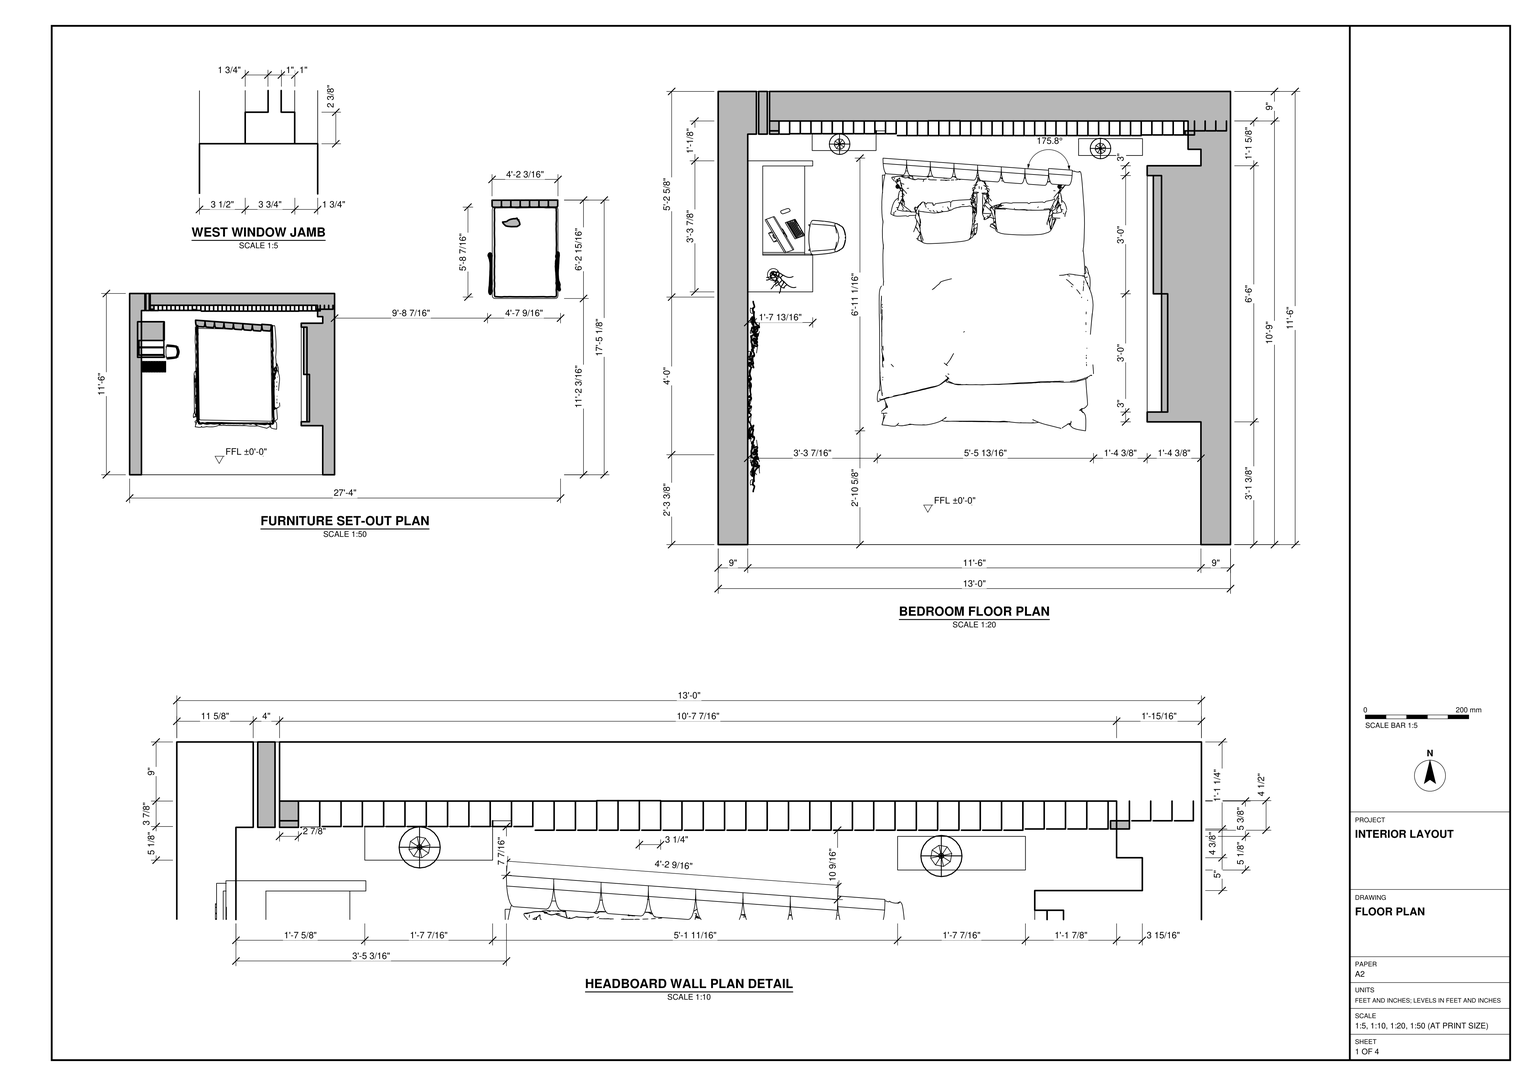
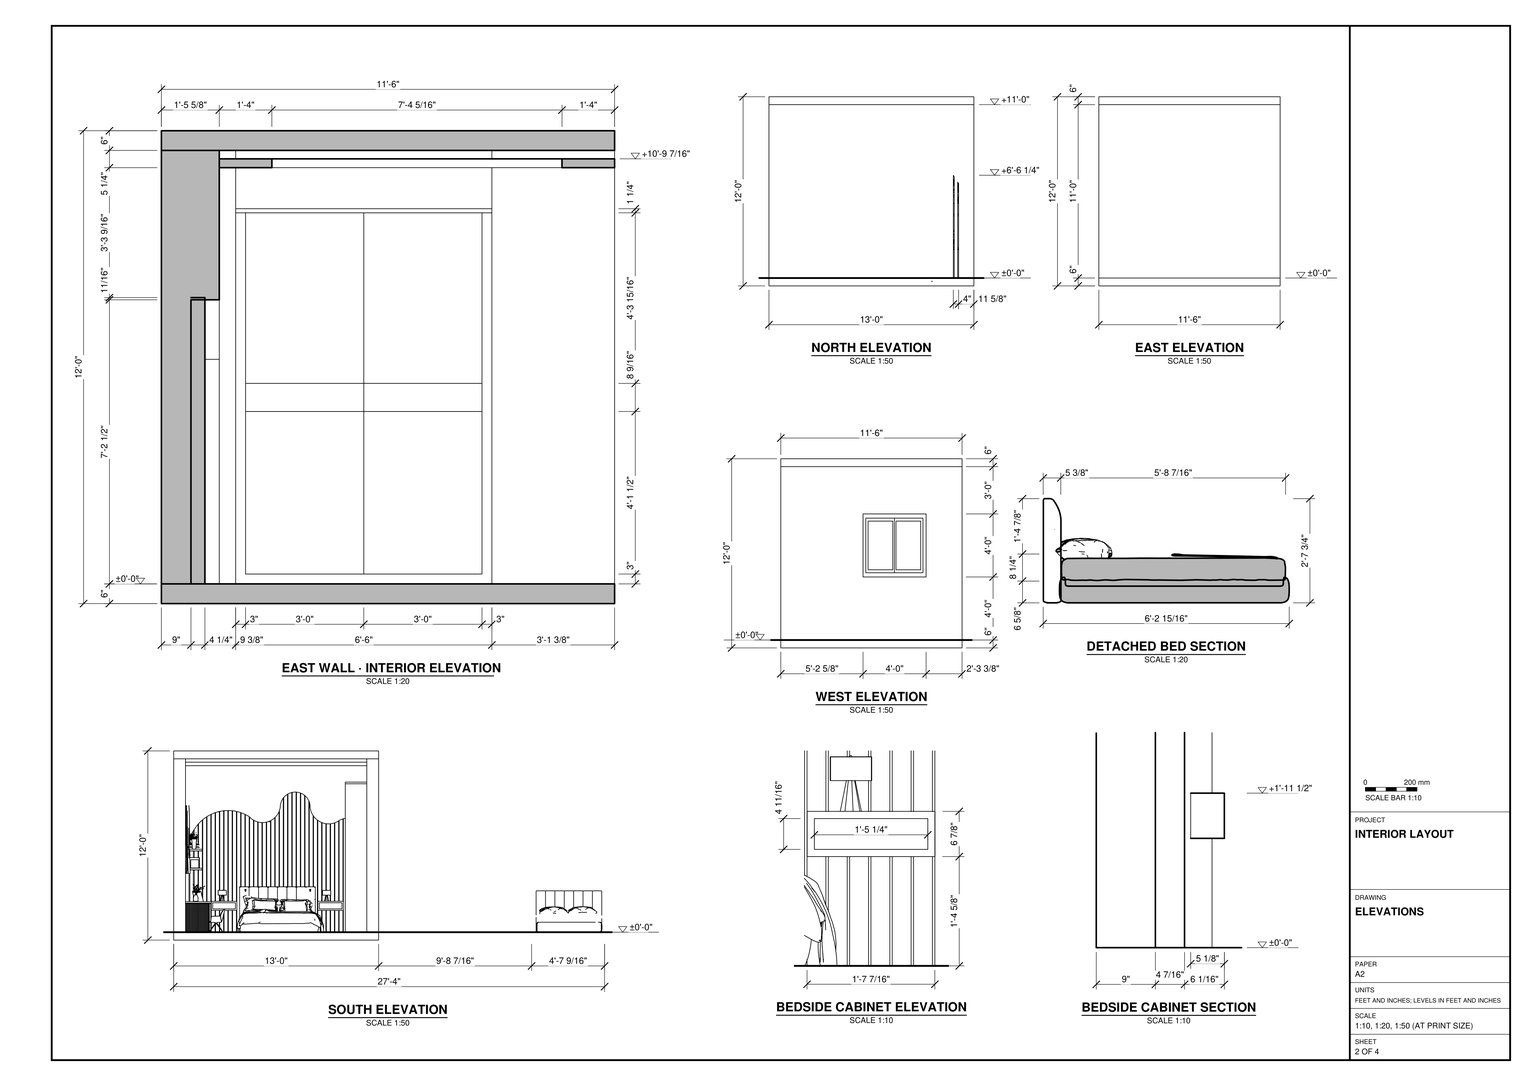
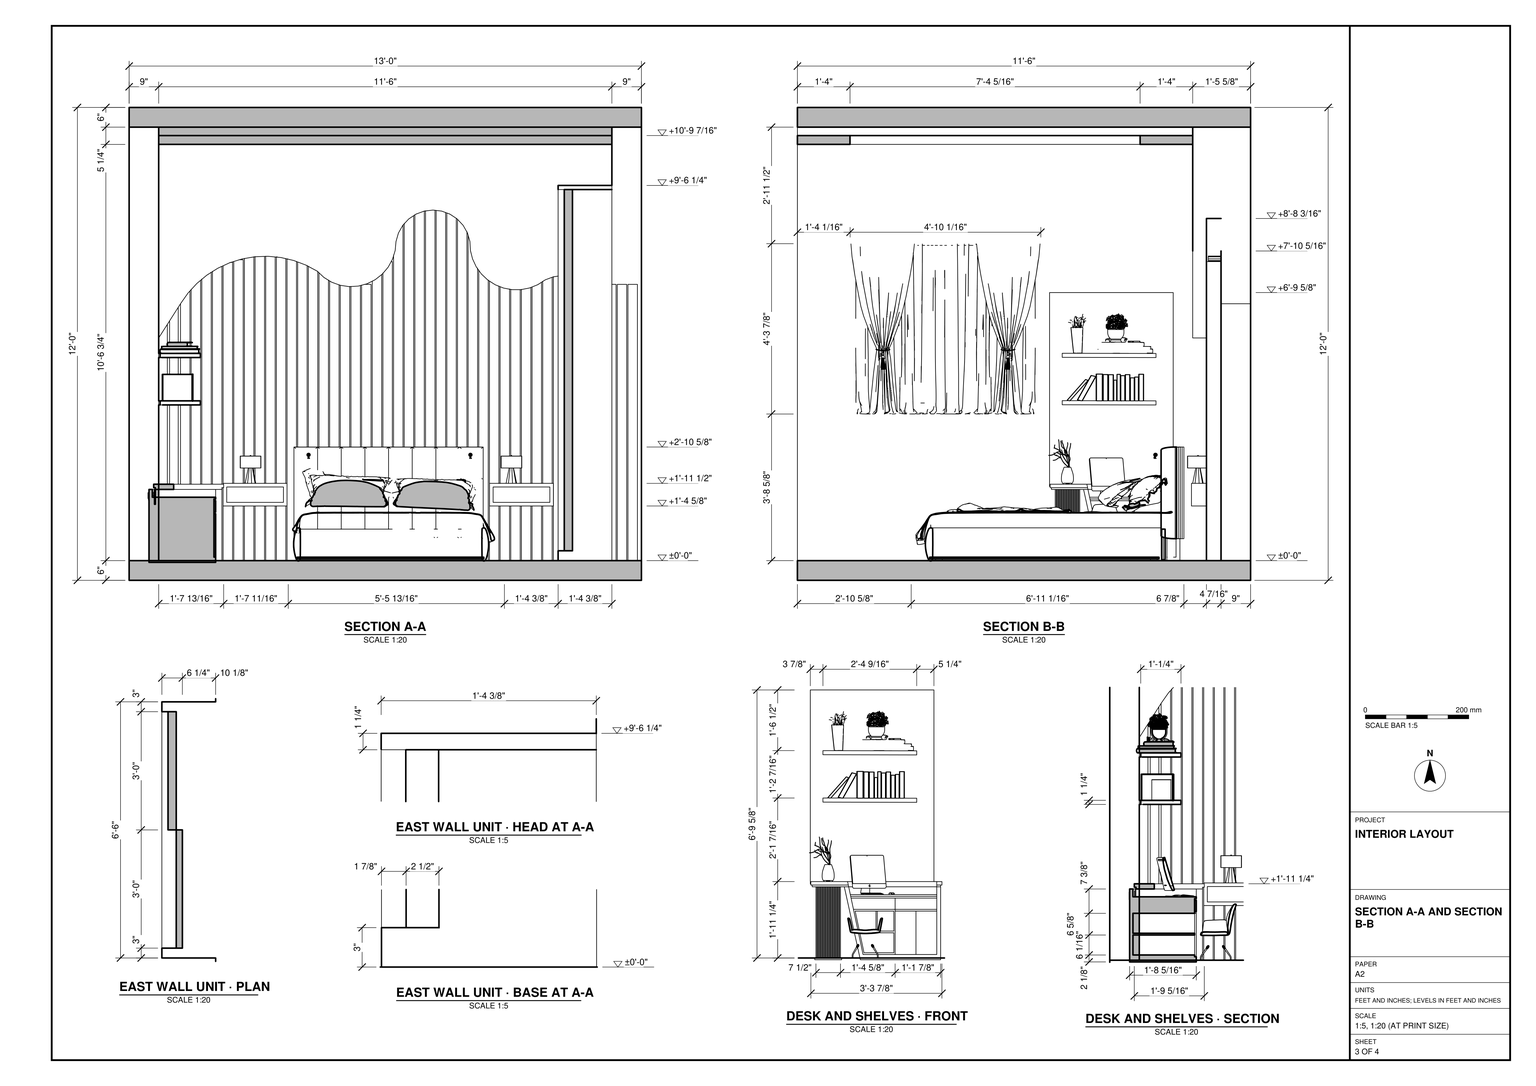
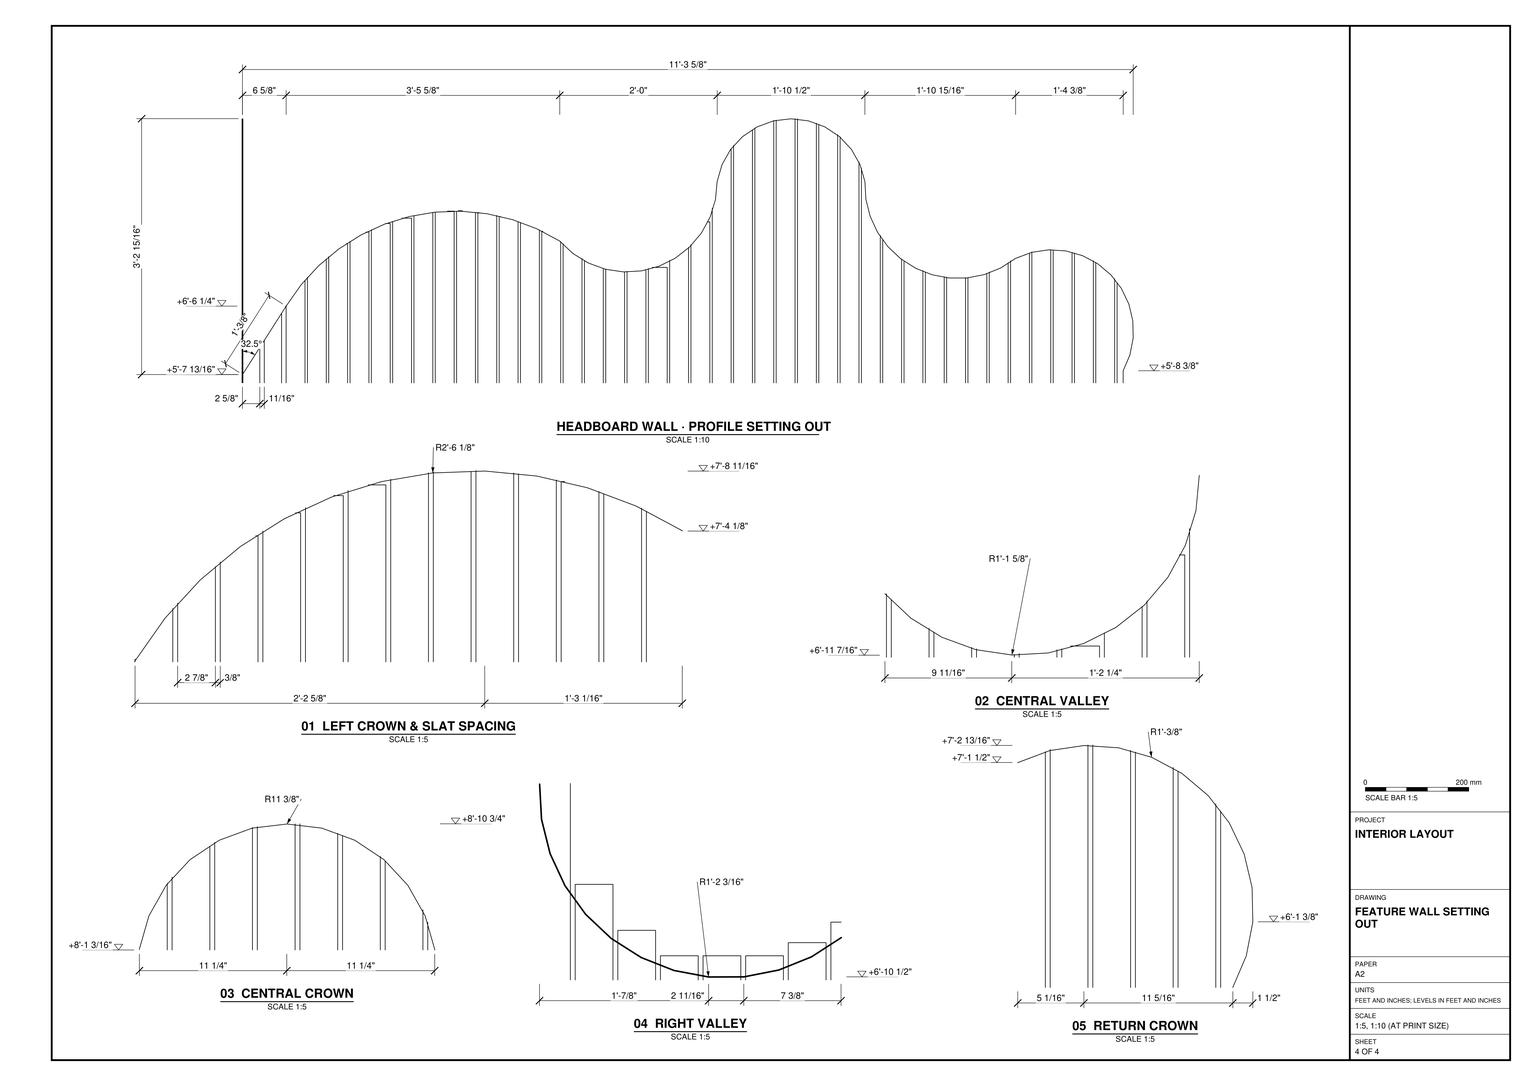
Build the bedroom in SketchUp from task_files/diagram_01.pdf. Work in feet and inches, with the finished floor at ±0'-0". The complete set-out, including the detached bed, measures 27'-4" along X, 17'-5 1/8" along Y and 12'-0" along Z. Do not use these overall dimensions as the room footprint: the bedroom shell is 13'-0" wide by 11'-6" deep.

Model the floor and ceiling slabs and the north, east and west walls at the thicknesses shown. Leave the south side open as in the south elevation. Form the framed window opening in the west wall and place the desk, chair and wall shelves near the head of the bed. On the north wall, form the varying heights of the vertical slats to match the curved upper edge in section A-A. Set the main bed at the slight angle shown in plan, with a raised bedside cabinet on either side. Build the projecting east wall unit with its paired fronts, head and base. Include the smaller detached bed outside the room at the offset shown on the furniture set-out plan.

Decor and loose items, including lamps, plants, books and cushions, may be any suitable library components placed where shown. Keep shell elements and individual furniture and joinery pieces in separate groups or components, and use components for repeated parts. Save one SketchUp model as output_files/bedroom_fit_out_and_detached_bed.skp.

# SketchUp Ruby script. Lengths in inches.
U = 1.inch
M = Sketchup.active_model
def pt(a) = Geom::Point3d.new(a.map { |v| v * U })
def face(e, loops, mat)
  f = e.add_face(loops[0].map { |a| pt(a) })
  loops[1..].each { |l| e.add_face(l.map { |a| pt(a) }).erase! }
  f.material = f.back_material = mat if mat
  f
end
# faces: each face lists its corners as indices into pts; further lists are holes
def faces(e, pts, list, mat = nil) = list.each { |f| face(e, (f[0].is_a?(Array) ? f : [f]).map { |l| l.map { |i| pts[i] } }, mat) }
# xy, xz, yz: faces in a plane at the given z, y or x. An outline is a flat list of corners, or four numbers for a rectangle; further outlines are holes
def ring(l) = l.size == 4 ? [[l[0], l[1]], [l[2], l[1]], [l[2], l[3]], [l[0], l[3]]] : l.each_slice(2).to_a
def flat(e, list, mat, &to3) = list.each { |f| face(e, (f[0].is_a?(Array) ? f : [f]).map { |l| ring(l).map { |u, v| to3.(u, v) } }, mat) }
def xy(e, z, list, mat = nil) = flat(e, list, mat) { |x, y| [x, y, z] }
def xz(e, y, list, mat = nil) = flat(e, list, mat) { |x, z| [x, y, z] }
def yz(e, x, list, mat = nil) = flat(e, list, mat) { |y, z| [x, y, z] }
def lines(e, pts, list) = list.each { |a, b| e.add_line(pt(pts[a]), pt(pts[b])) }
# prism: a flat outline (further loops are holes) pulled along v
def prism(e, loops, v, mat = nil)
  f = face(e, loops, mat); d = Geom::Vector3d.new(v.map { |x| x * U })
  f.pushpull(f.normal.samedirection?(d) ? d.length : -d.length)
end
def box(e, o, s, mat = nil) = prism(e, [[o, [o[0] + s[0], o[1], o[2]], [o[0] + s[0], o[1] + s[1], o[2]], [o[0], o[1] + s[1], o[2]]]], [0, 0, s[2]], mat)
def at(x, y, z, deg = 0) = Geom::Transformation.translation(pt([x, y, z])) * Geom::Transformation.rotation(ORIGIN, Z_AXIS, deg.degrees)
def axes(o, x, y, z) = Geom::Transformation.new([*x, 0, *y, 0, *z, 0, *pt(o).to_a, 1])
def part(name) = M.definitions.add(name)
# library, detail: a bought-in or finely detailed component or shape, given as its bounding box
def library(name, o, s) = part(name).tap { |d| box(d.entities, o, s) }
def detail(e, o, s) = box(e.add_group.entities, o, s)
def put(e, d, t, mat = nil) = e.add_instance(d, t).tap { |i| i.material = mat if mat }
def group(e, t, mat = nil) = e.add_group.tap { |g| g.transformation = t; g.material = mat if mat }.entities
root = M.entities
M.materials.add("Material__1").color = [51, 42, 44]
M.materials.add("Material__2").color = [97, 132, 37]
M.materials.add("[Color A02]").color = [255, 153, 153]
M.materials.add("[Color B01]").color = [255, 216, 204]
M.materials.add("[Translucent_Glass_Safety]").color = [204, 235, 244]
M.materials["[Translucent_Glass_Safety]"].alpha = 0.5
M.materials.add("[Translucent_Glass_Sky_Reflection]").color = [125, 138, 183]
M.materials["[Translucent_Glass_Sky_Reflection]"].alpha = 0.52
M.materials.add("[Wood Bamboo]").color = [177, 105, 43]
c1 = library("BED+3",[-244.73,-59.6875,196.6875],[91.01,69.4,39.64])
c2 = library("Group14",[-64.97,9.24,0.31],[138.52,9.93,292.57])
c3 = library("Group16",[86.37,-10.76,76.46],[21.79,14.87,35.97])
c4 = library("Group22",[48.82,-10.91,0.23],[97.72,18.57,293.12])
c5 = library("Group24",[44.03,2.01,0.26],[103.73,11,292.35])
c6 = library("Group27",[-106.21,-10.76,76.46],[21.8,14.87,35.97])
c7 = library("Group35",[-145.81,2.01,0.26],[103.73,11,292.35])
c8 = library("Group33",[-144.59,-10.91,0.23],[97.72,18.57,293.12])
c9 = part("rem")
g1 = group(c9.entities,at(-145.81,-10.91,0.23))
put(g1,c2,at(145.81,10.91,-0.23))
put(g1,c3,at(145.81,10.91,-0.23))
put(g1,c4,at(145.81,10.91,-0.23))
put(g1,c5,at(145.81,10.91,-0.23))
put(g1,c6,at(145.81,10.91,-0.23))
put(g1,c7,at(145.81,10.91,-0.23))
put(g1,c8,at(145.81,10.91,-0.23))
c10 = part("Two-panel window")
xy(c10.entities,0,[[0,0,4.33,55.51]])
xy(c10.entities,2.76,[[0,2.76,2,27.76],[3.15,2.76,4.33,27.76],[0,27.76,0.82,52.76],[0.82,27.76,2.36,52.76],[2.36,27.76,4.33,52.76]])
xy(c10.entities,4.72,[[2,4.72,2.4,26.38],[2.76,4.72,3.15,26.38],[0.82,29.13,1.22,50.79],[1.97,29.13,2.36,50.79]])
xy(c10.entities,36.61,[[2,4.72,2.4,26.38],[2.76,4.72,3.15,26.38],[0.82,29.13,1.22,50.79],[1.97,29.13,2.36,50.79]])
xy(c10.entities,38.58,[[0,2.76,2,27.76],[3.15,2.76,4.33,27.76],[0,27.76,0.82,52.76],[0.82,27.76,2.36,52.76],[2.36,27.76,4.33,52.76]])
xy(c10.entities,41.34,[[0,0,4.33,55.51]])
xz(c10.entities,0,[[0,0,4.33,41.34]])
xz(c10.entities,2.76,[[0,2.76,2,38.58],[3.15,2.76,4.33,38.58]])
xz(c10.entities,4.72,[[2,4.72,2.4,36.61],[2.76,4.72,3.15,36.61]])
xz(c10.entities,26.38,[[2,4.72,2.4,36.61],[2.76,4.72,3.15,36.61]])
xz(c10.entities,27.76,[[0.82,2.76,2,38.58],[2,2.76,2.36,38.58],[2.36,2.76,3.15,38.58]])
xz(c10.entities,29.13,[[0.82,4.72,1.22,36.61],[1.97,4.72,2.36,36.61]])
xz(c10.entities,50.79,[[0.82,4.72,1.22,36.61],[1.97,4.72,2.36,36.61]])
xz(c10.entities,52.76,[[0,2.76,0.82,38.58],[0.82,2.76,2.36,38.58],[2.36,2.76,4.33,38.58]])
xz(c10.entities,55.51,[[0,0,4.33,41.34]])
yz(c10.entities,0,[[[0,0,55.51,41.34],[2.76,2.76,52.76,38.58]]])
yz(c10.entities,0.82,[[[27.76,2.76,52.76,38.58],[29.13,4.72,50.79,36.61]]])
yz(c10.entities,1.22,[[29.13,4.72,50.79,36.61]],"[Translucent_Glass_Sky_Reflection]")
yz(c10.entities,1.97,[[29.13,4.72,50.79,36.61]],"[Translucent_Glass_Sky_Reflection]")
yz(c10.entities,2,[[[2.76,2.76,27.76,38.58],[4.72,4.72,26.38,36.61]]])
yz(c10.entities,2.36,[[[27.76,2.76,52.76,38.58],[29.13,4.72,50.79,36.61]]])
yz(c10.entities,2.4,[[4.72,4.72,26.38,36.61]],"[Translucent_Glass_Safety]")
yz(c10.entities,2.76,[[4.72,4.72,26.38,36.61]],"[Translucent_Glass_Safety]")
yz(c10.entities,3.15,[[[2.76,2.76,27.76,38.58],[4.72,4.72,26.38,36.61]]])
yz(c10.entities,4.33,[[[0,0,55.51,41.34],[2.76,2.76,52.76,38.58]]])
c11 = library("Lamp+10 (1)",[0,0,0],[16.92,16.92,22.79])
c12 = library("LIVROS\#1",[1.04,0,0],[11.9,15.35,3.36])
c13 = library("Grupo\#1",[-43.96,137.13,0],[1211.05,2538.28,152.47])
c14 = part("APPLE IPHONE 5S")
put(c14.entities,c13,at(0,0,0))
c15 = part("iPhone 5s Cinza Espacial")
put(c15.entities,c14,at(0,0,0))
c16 = part("iPhone 5s Prateado")
put(c16.entities,c15,at(0,0,0))
c17 = library("OCULOS1",[0,0,0],[5.82,6.14,1.45])
c18 = library("Group145\#1",[5.875,6.46,9.56],[20.8,10.13,11.36])
c19 = library("\#1",[-138.85,-135.75,0],[277.7,270.97,9.64])
c20 = library("\#2",[-34.84,-73.35,-33.91],[69.68,146.26,68.31])
c21 = library("\#5",[-4127.85,-1300.75,-2324.72],[5349.84,4521.24,5423.31])
c22 = part("\#3\#1")
put(c22.entities,c21,at(450.18,-1111.4375,0),"Material__2")
c23 = part("12")
put(c23.entities,c19,axes([-49.79,-36.9375,349.64],[0.59279,0,0],[0,0.59279,0],[0,0,0.59279]),"Material__1")
put(c23.entities,c20,axes([-39.24,-18.18,177.19],[1.20819,-2.09264,0],[0,0,2.41638],[2.09264,1.20819,0]))
put(c23.entities,c22,axes([-83.44,-46.04,442.44],[-0.03636,-0.03293,-0.01473],[-0.00083,-0.02391,0.05549],[0.02997,-0.02791,-0.01158]))
c24 = library("Sphere Light",[-1.84,-1.84,-1.84],[3.68,3.68,3.68])
c25 = library("Sphere Light\#1",[-1.95,-1.95,-1.95],[3.9,3.9,3.9])
c26 = part("Group\#3")
xy(c26.entities,84.125,[[0,0,2.875,3]])
xz(c26.entities,0,[[0,0,2.875,84.125]])
yz(c26.entities,2.875,[[0,0,3,84.125]])
c27 = library("Group\#4",[-2.46,-2.1,0],[81.3,95.2,42.26])
c28 = library("Group\#49",[0,-1.12,0],[35.56,82.36,58.48])
c29 = library("Group",[-10.56,-10.46,-0.01],[21.3,22.85,34.81])
c30 = library("Agrupar\#111",[0,0,0],[6.57,6.6875,8.75])
xy(root,-6,[[0,0,156,138]],"[Color B01]")
xy(root,0,[[0,0,9,0,9,125,11.63,125,11.63,138,0,138],[9,0,147,0,147,37.375,130.625,37.375,130.625,115.375,147,115.375,147,120.375,143.08,120.375,143.08,124.75,142.16,124.75,142.16,126,143.08,126,143.08,129,73.67,129,73.67,129.0625,63.93,129.0625,63.93,129,18.52,129,18.52,125,15.64,125,15.64,138,14.95,138,14.95,125,12.32,125,12.32,138,11.63,138,11.63,125,9,125],[147,0,156,0,156,138,15.64,138,15.64,129,63.93,129,63.93,129.0625,73.67,129.0625,73.67,129,143.08,129,143.08,126,145.03,126,145.03,124.75,143.08,124.75,143.08,120.375,147,120.375,147,115.375,130.625,115.375,130.625,37.375,147,37.375],[142.16,124.75,143.08,126],[143.08,124.75,145.03,126],
  [12.32,125,14.95,138],[15.64,125,18.52,129],[48.08,125.125,50.96,126]],"[Color B01]")
xy(root,3,[[130.625,40.375,135,40.375,135,76.375,132.5,76.375,132.5,112.375,130.625,112.375],[135,40.375,136.875,76.375],[132.5,76.375,135,112.375]],"[Color B01]")
xy(root,16.64,[[109.74,118.5,129.21,123.625]])
xy(root,16.64,[[28.62,120,48.08,125.125]],"[Color B01]")
xy(root,23.53,[[109.74,118.5,129.21,123.625]])
xy(root,23.53,[[28.62,120,48.08,125.125]],"[Color B01]")
xy(root,48,[[0,27.375,9,27.375,9,73.63,0,75.375]],"[Color B01]")
xy(root,84.125,[[64.3,124.5625,67.18,129],[67.55,124.5625,70.42,129],[70.79,124.5625,73.67,129],[112.96,124.5625,115.84,129],[116.21,124.5625,119.08,129],
  [119.45,124.5625,122.33,129],[142.16,124.75,145.03,129],[15.64,125,18.52,129],[71.74,129,73.67,129.0625]],"[Color B01]")
xy(root,85.125,[[122.7,124.5625,125.57,129]],"[Color B01]")
xy(root,85.3125,[[61.06,124.5625,63.93,129],[138.92,124.75,141.79,129]],"[Color B01]")
xy(root,86.0625,[[109.72,124.5625,112.59,129]],"[Color B01]")
xy(root,86.625,[[135.67,124.75,138.55,129]],"[Color B01]")
xy(root,86.6875,[[125.9375,124.5625,128.8125,129]],"[Color B01]")
xy(root,87.1875,[[129.18,124.75,132.06,129]],"[Color B01]")
xy(root,87.25,[[74.03,124.5625,76.91,129]],"[Color B01]")
xy(root,87.75,[[22.13,125.125,25.01,129]],"[Color B01]")
xy(root,87.875,[[57.8125,124.5625,60.6875,129]],"[Color B01]")
xy(root,88,[[132.43,124.75,135.3,129]],"[Color B01]")
xy(root,88.4375,[[18.89,125,21.76,128.875]])
xy(root,89.5,[[25.375,125.125,28.25,129]],"[Color B01]")
xy(root,89.5625,[[106.48,124.5625,109.35,129]],"[Color B01]")
xy(root,89.625,[[54.57,124.5625,57.45,129]],"[Color B01]")
xy(root,90.8125,[[28.62,125.125,31.49,129]],"[Color B01]")
xy(root,91.0625,[[77.28,124.5625,80.15,129]],"[Color B01]")
xy(root,91.25,[[51.33,125.125,54.2,129]],"[Color B01]")
xy(root,91.375,[[48.08,126,50.96,129]],"[Color B01]")
xy(root,91.625,[[31.86,125.125,34.74,129]],"[Color B01]")
xy(root,91.875,[[48.08,125.125,50.96,129]],"[Color B01]")
xy(root,92.5,[[44.84,125.125,47.71,129]],"[Color B01]")
xy(root,92.625,[[35.11,125.125,37.98,129]],"[Color B01]")
xy(root,92.6875,[[38.35,125.125,41.23,129]],"[Color B01]")
xy(root,92.75,[[41.59,125.125,44.47,129]],"[Color B01]")
xy(root,96,[[0,27.375,0,75.375,9,73.63,9,27.375]],"[Color B01]")
xy(root,100.375,[[103.23,124.5625,106.11,129]],"[Color B01]")
xy(root,104.1875,[[80.52,124.5625,83.4,129]],"[Color B01]")
xy(root,104.6875,[[99.99,124.5625,102.86,129]],"[Color B01]")
xy(root,106.75,[[83.77,124.5625,86.64,129]],"[Color B01]")
xy(root,107.4375,[[96.74,124.5625,99.62,129]],"[Color B01]")
xy(root,107.875,[[87.01,124.5625,89.89,129]],"[Color B01]")
xy(root,108.25,[[93.5,124.5625,96.375,129]],"[Color B01]")
xy(root,108.75,[[90.25,124.5625,93.13,129]],"[Color B01]")
xy(root,113,[[130.625,37.375,147,40.375],[135,40.375,136.875,76.375],[136.875,40.375,147,76.375],[132.5,76.375,135,112.375],[132.5,76.375,135,112.375],
  [135,76.375,147,112.375],[130.625,112.375,147,115.375]],"[Color B01]")
xy(root,114.25,[[130.625,37.375,147,115.375]],"[Color B01]")
xy(root,126.75,[[[9,0,147,120.375],[25.02,16.02,130.98,104.36]]])
xy(root,129.4375,[[[9,0,147,120.375],[25.02,16.02,130.98,104.36]],[25.02,16.02,130.98,104.36]])
xy(root,132,[[9,0,147,120.375]])
xy(root,132,[[0,0,0,138,156,138,156,0,147,0,147,120.375,9,120.375,9,0]],"[Color B01]")
xy(root,138,[[0,0,156,138]])
xz(root,0,[[9,126.75,147,129.4375],[0,132,156,138]])
xz(root,0,[[0,-6,156,0],[0,0,9,132],[147,0,156,132]],"[Color B01]")
xz(root,16.02,[[25.02,126.75,130.98,129.4375]])
xz(root,27.375,[[0,48,9,96]],"[Color B01]")
xz(root,37.375,[[130.625,0,147,113],[130.625,113,147,114.25]],"[Color B01]")
xz(root,40.375,[[130.625,3,135,113],[135,3,136.875,113]],"[Color B01]")
xz(root,76.375,[[132.5,3,135,113],[135,3,136.875,113]],"[Color B01]")
xz(root,80.64,[[9,47.47,9.4375,48.72],[9.4375,47.47,21.6875,48.72],[9,61.9,9.4375,63.15],[9.4375,61.9,21.6875,63.15]],"[Wood Bamboo]")
xz(root,109.2,[[9,47.4,9.4375,48.65],[9,61.84,9.4375,63.09]],"[Color B01]")
xz(root,109.2,[[9.4375,47.4,21.6875,48.65],[9.4375,61.84,21.6875,63.09]],"[Wood Bamboo]")
xz(root,112.375,[[130.625,3,132.5,113],[132.5,3,135,113]],"[Color B01]")
xz(root,115.375,[[130.625,0,147,113],[130.625,113,147,114.25]],"[Color B01]")
xz(root,118.5,[[[109.74,16.64,129.21,23.53],[110.84,17.74,128.11,22.43]],[110.84,17.74,128.11,22.43]])
xz(root,120,[[[28.62,16.64,48.08,23.53],[29.71,17.74,46.99,22.43]],[29.71,17.74,46.99,22.43]],"[Color B01]")
xz(root,120.375,[[9,126.75,147,129.4375]])
xz(root,120.375,[[143.08,0,147,0,147,126.75,9,126.75,9,67.8125,15.64,78.23,17.92,81.47,20.61,84.39,23.65,86.93,27.01,89.05,30.61,90.7,34.4,91.875,38.31,92.54,42.27,92.68,46.22,92.3,50.08,91.41,53.79,90.01,57.29,88.14,59.3,86.25,61.66,84.79,64.26,83.85,67,83.44,69.76,83.6,72.43,84.31,74.91,85.54,77.09,87.25,78.875,89.36,80.2,91.79,81.01,94.4375,81.26,97.19,82,99.76,83.3125,102.09,85.13,104.04,87.36,105.52,89.86,106.44,92.51,106.76,95.17,106.44,97.67,105.52,99.9,104.04,101.72,102.09,103.03,99.76,103.76,97.19,103.91,94.51,104.5625,91.9,105.69,89.46,107.27,87.28,109.22,85.4375,111.49,84,113.99,83.01,116.63,82.51,119.32,82.52,121.96,83.04,124.45,84.04,126.71,85.5,129.16,86.42,131.76,86.81,134.375,86.63,136.9,85.92,139.21,84.68,141.22,82.99,142.82,80.91,143.95,78.55,144.55,76,144.61,73.375,144.11,70.8,143.08,68.39],[9,129.4375,147,132]],"[Color A02]")
xz(root,124.5625,[[54.57,0,57.45,89.625],[57.8125,0,60.6875,87.875],[61.06,0,63.93,85.3125],[64.3,0,67.18,84.125],[67.55,0,70.42,84.125],
  [70.79,0,73.67,84.125],[74.03,0,76.91,87.25],[77.28,0,80.15,91.0625],[80.52,0,83.4,104.1875],[83.77,0,86.64,106.75],
  [87.01,0,89.89,107.875],[90.25,0,93.13,108.75],[93.5,0,96.375,108.25],[96.74,0,99.62,107.4375],[99.99,0,102.86,104.6875],
  [103.23,0,106.11,100.375],[106.48,0,109.35,89.5625],[109.72,0,112.59,86.0625],[112.96,0,115.84,84.125],[116.21,0,119.08,84.125],
  [119.45,0,122.33,84.125],[122.7,0,125.57,85.125],[125.9375,0,128.8125,86.6875]],"[Color B01]")
xz(root,124.75,[[129.18,0,132.06,87.1875],[132.43,0,135.3,88],[135.67,0,138.55,86.625],[138.92,0,141.79,85.3125],[142.16,0,145.03,84.125]],"[Color B01]")
xz(root,125,[[9,0,11.63,0,11.63,71.94,9,67.8125],[12.32,0,14.95,0,14.95,77.15,12.32,73.02],[15.64,0,18.52,84.125],[18.89,0,21.76,88.4375]],"[Color B01]")
xz(root,125.125,[[22.13,0,25.01,87.75],[25.375,0,28.25,89.5],[28.62,0,31.49,16.64],[31.86,0,34.74,16.64],[35.11,0,37.98,16.64],
  [38.35,0,41.23,16.64],[41.59,0,44.47,16.64],[44.84,0,47.71,16.64],[48.08,0,50.96,91.875],[51.33,0,54.2,91.25],
  [28.62,16.64,31.49,23.53],[31.49,16.64,31.86,23.53],[31.86,16.64,34.74,23.53],[34.74,16.64,35.11,23.53],[35.11,16.64,37.98,23.53],
  [37.98,16.64,38.35,23.53],[38.35,16.64,41.23,23.53],[41.23,16.64,41.59,23.53],[41.59,16.64,44.47,23.53],[44.47,16.64,44.84,23.53],
  [44.84,16.64,47.71,23.53],[47.71,16.64,48.08,23.53],[28.62,23.53,31.49,90.8125],[31.86,23.53,34.74,91.625],[35.11,23.53,37.98,92.625],
  [38.35,23.53,41.23,92.6875],[41.59,23.53,44.47,92.75],[44.84,23.53,47.71,92.5]],"[Color B01]")
xz(root,126,[[15.64,0,18.52,84.125],[142.16,0,145.03,84.125]],"[Color B01]")
xz(root,129,[[15.64,0,18.52,0,18.52,82.12,17.92,81.47,15.64,78.23],[18.52,0,25.01,0,25.01,87.75,24.95,87.75,23.65,86.93,20.61,84.39,18.52,82.12],[25.01,0,28.25,0,28.25,89.5,27.99,89.5,27.01,89.05,24.95,87.75,25.01,87.75],[28.25,0,31.49,0,31.49,90.8125,30.96,90.8125,30.61,90.7,27.99,89.5,28.25,89.5],[31.49,0,34.74,0,34.74,91.625,33.59,91.625,30.96,90.8125,31.49,90.8125],
  [34.74,0,37.98,0,37.98,92.48,34.4,91.875,33.59,91.625,34.74,91.625],[37.98,0,41.23,0,41.23,92.64,38.31,92.54,37.98,92.48],[41.23,0,44.47,0,44.47,92.47,42.27,92.68,41.23,92.64],[44.47,0,47.71,0,47.71,91.96,46.22,92.3,44.47,92.47],[47.71,0,50.96,0,50.96,91.08,50.17,91.375,48.08,91.375,48.08,91.87,47.71,91.96],
  [50.96,0,54.2,0,54.2,89.8,53.79,90.01,50.96,91.08],[54.2,0,57.45,0,57.45,88,57.29,88.14,56.04,88.8125,54.57,88.8125,54.57,89.6,54.2,89.8],[57.45,0,60.6875,0,60.6875,85.39,59.3,86.25,58.9,86.625,57.8125,86.625,57.8125,87.65,57.45,88],[60.6875,0,63.93,0,63.93,83.97,63.5,84.125,61.06,84.125,61.06,85.16,60.6875,85.39],[73.67,0,76.91,0,76.91,87.11,74.91,85.54,72.43,84.31,71.74,84.125,73.67,84.125],
  [76.91,0,80.15,0,80.15,91.0625,79.8,91.0625,78.875,89.36,77.09,87.25,76.91,87.11],[80.15,0,83.4,0,83.4,102.18,83.3125,102.09,82,99.76,81.26,97.19,81.01,94.4375,80.2,91.79,79.8,91.0625,80.15,91.0625],[83.4,0,86.64,0,86.64,105.05,85.13,104.04,83.4,102.18],[86.64,0,89.89,0,89.89,106.45,89.86,106.44,87.36,105.52,86.64,105.05],[89.89,0,93.13,0,93.13,106.68,92.51,106.76,89.89,106.45],
  [93.13,0,96.375,0,96.375,106,95.17,106.44,93.13,106.68],[96.375,0,99.62,0,99.62,104.23,97.67,105.52,96.375,106],[99.62,0,102.86,0,102.86,100.05,101.72,102.09,99.9,104.04,99.62,104.23],[102.86,0,106.11,0,106.11,88.89,105.69,89.46,104.5625,91.9,103.91,94.51,103.76,97.19,103.03,99.76,102.86,100.05],[106.11,0,109.35,0,109.35,85.36,109.22,85.4375,107.27,87.28,106.11,88.89],
  [109.35,0,112.59,0,112.59,83.5625,111.49,84,111.29,84.125,109.72,84.125,109.72,85.12,109.35,85.36],[112.59,0,115.84,0,115.84,82.66,113.99,83.01,112.59,83.5625],[115.84,0,119.08,0,119.08,82.52,116.63,82.51,115.84,82.66],[119.08,0,122.33,0,122.33,83.1875,121.96,83.04,119.32,82.52,119.08,82.52],[122.33,0,125.57,0,125.57,84.125,124.58,84.125,124.45,84.04,122.33,83.1875],
  [125.57,0,128.8125,0,128.8125,86.29,126.71,85.5,125.57,84.77],[128.8125,0,132.06,0,132.06,86.79,131.76,86.81,129.16,86.42,128.8125,86.29],[132.06,0,135.3,0,135.3,86.37,134.375,86.63,132.06,86.79],[135.3,0,138.55,0,138.55,85.04,136.9,85.92,135.3,86.37],[138.55,0,141.79,0,141.79,82.25,141.22,82.99,139.87,84.125,138.92,84.125,138.92,84.84,138.55,85.04],
  [141.79,0,143.08,0,143.08,68.39,144.11,70.8,144.61,73.375,144.55,76,143.95,78.55,142.82,80.91,141.79,82.25],[61.06,84.125,63.5,84.125,61.66,84.79,61.06,85.16],[63.5,84.125,61.66,84.79,61.06,85.16,61.06,85.3125,63.5,85.3125],[63.5,84.125,63.93,85.3125],[109.72,84.125,111.29,84.125,109.72,85.12],
  [111.29,84.125,109.72,85.12,109.72,86.0625,111.29,86.0625],[111.29,84.125,112.59,86.0625],[122.7,84.125,124.58,85.125],[124.58,84.125,124.58,85.125,125.57,85.125,125.57,84.77],[124.58,84.125,125.57,84.125,125.57,84.77],
  [138.92,84.125,139.87,84.125,139.21,84.68,138.92,84.84],[139.87,84.125,139.21,84.68,138.92,84.84,138.92,85.3125,139.87,85.3125],[139.87,84.125,141.79,85.3125],[57.8125,86.625,58.9,86.625,58.17,87.3125,57.8125,87.3125],[58.9,86.625,58.17,87.3125,58.9,87.3125],
  [58.9,86.625,60.6875,87.3125],[57.8125,87.3125,58.17,87.3125,57.8125,87.65],[58.17,87.3125,57.8125,87.65,57.8125,87.875,58.17,87.875],[58.17,87.3125,58.9,87.875],[58.9,87.3125,60.6875,87.875],
  [54.57,88.8125,54.57,89.6,56.04,88.8125],[54.57,88.8125,56.04,88.8125,54.57,89.6],[56.04,88.8125,54.57,89.6,54.57,89.625,56.04,89.625],[56.04,88.8125,57.45,89.625],[48.08,91.375,48.08,91.87,50.08,91.41,50.17,91.375],
  [48.08,91.375,50.17,91.375,50.08,91.41,48.08,91.87],[50.17,91.375,50.08,91.41,48.08,91.87,48.08,91.875,50.17,91.875],[50.17,91.375,50.96,91.875]],"[Color B01]")
xz(root,129.0625,[[63.93,0,73.67,0,73.67,84.125,71.74,84.125,69.76,83.6,67,83.44,64.26,83.85,63.93,83.97]],"[Color B01]")
xz(root,138,[[0,132,156,138]])
xz(root,138,[[0,-6,156,0],[0,0,0,132,156,132,156,0,15.64,0,15.64,78.23,14.95,77.15,14.95,0,12.32,0,12.32,73.02,11.63,71.94,11.63,0]],"[Color B01]")
yz(root,0,[[0,132,138,138]])
yz(root,0,[[0,-6,138,0],[[0,0,138,132],[27.375,48,75.375,96]]],"[Color B01]")
yz(root,9,[[0,126.75,120.375,129.4375]])
yz(root,9,[[[0,0,125,0,125,67.8125,120.375,67.8125,120.375,126.75,0,126.75],[76.79,22.5625,114.4375,81.625],[27.375,48,73.63,96]],[0,129.4375,120.375,132]],"[Color B01]")
yz(root,9,[[[76.79,22.5625,114.4375,81.625],[109.2,47.4,80.64,47.47,80.64,48.72,109.2,48.65],[109.2,61.84,80.64,61.9,80.64,63.15,109.2,63.09]]],"[Wood Bamboo]")
yz(root,9.4375,[[109.2,47.4,80.64,47.47,80.64,48.72,109.2,48.65],[109.2,61.84,80.64,61.9,80.64,63.15,109.2,63.09]],"[Color B01]")
yz(root,11.63,[[125,0,138,71.94]],"[Color B01]")
yz(root,12.32,[[125,0,138,73.02]],"[Color B01]")
yz(root,14.95,[[125,0,138,77.15]],"[Color B01]")
yz(root,15.64,[[125,0,126,78.23],[126,0,129,78.23],[129,0,138,78.23],[125,78.23,126,84.125]],"[Color B01]")
yz(root,18.52,[[125,0,129,84.125]],"[Color B01]")
yz(root,21.6875,[[109.2,47.4,109.2,48.65,80.64,48.72,80.64,47.47],[109.2,61.84,109.2,63.09,80.64,63.15,80.64,61.9]],"[Wood Bamboo]")
yz(root,21.76,[[125,0,128.875,88.4375]],"[Color B01]")
yz(root,25.01,[[125.125,0,129,87.75]],"[Color B01]")
yz(root,28.25,[[125.125,0,129,89.5]],"[Color B01]")
yz(root,28.62,[[120,16.64,125.125,23.53]],"[Color B01]")
yz(root,31.49,[[125.125,0,129,90.8125]],"[Color B01]")
yz(root,34.74,[[125.125,0,129,91.625]],"[Color B01]")
yz(root,37.98,[[125.125,0,129,92.625]],"[Color B01]")
yz(root,41.23,[[125.125,0,129,92.6875]],"[Color B01]")
yz(root,44.47,[[125.125,0,129,92.75]],"[Color B01]")
yz(root,47.71,[[125.125,0,129,92.5]],"[Color B01]")
yz(root,48.08,[[125.125,0,126,91.375],[120,16.64,125.125,23.53],[125.125,91.375,129,91.875]],"[Color B01]")
yz(root,50.96,[[125.125,0,129,91.375],[125.125,91.375,129,91.875]],"[Color B01]")
yz(root,54.2,[[125.125,0,129,91.25]],"[Color B01]")
yz(root,57.45,[[124.5625,0,129,88.8125],[124.5625,88.8125,129,89.625]],"[Color B01]")
yz(root,57.8125,[[124.5625,87.3125,129,87.875]],"[Color B01]")
yz(root,60.6875,[[124.5625,0,129,86.625],[124.5625,86.625,129,87.3125],[124.5625,87.3125,129,87.875]],"[Color B01]")
yz(root,63.93,[[124.5625,0,129,84.125],[129,0,129.0625,83.97],[124.5625,84.125,129,85.3125]],"[Color B01]")
yz(root,67.18,[[124.5625,0,129,84.125]],"[Color B01]")
yz(root,70.42,[[124.5625,0,129,84.125]],"[Color B01]")
yz(root,73.67,[[124.5625,0,129,84.125],[129,0,129.0625,84.125]],"[Color B01]")
yz(root,76.91,[[124.5625,0,129,87.25]],"[Color B01]")
yz(root,80.15,[[124.5625,0,129,91.0625]],"[Color B01]")
yz(root,83.4,[[124.5625,0,129,104.1875]],"[Color B01]")
yz(root,86.64,[[124.5625,0,129,106.75]],"[Color B01]")
yz(root,89.89,[[124.5625,0,129,107.875]],"[Color B01]")
yz(root,93.13,[[124.5625,0,129,108.75]],"[Color B01]")
yz(root,96.375,[[124.5625,0,129,108.25]],"[Color B01]")
yz(root,99.62,[[124.5625,0,129,107.4375]],"[Color B01]")
yz(root,102.86,[[124.5625,0,129,104.6875]],"[Color B01]")
yz(root,106.11,[[124.5625,0,129,100.375]],"[Color B01]")
yz(root,109.35,[[124.5625,0,129,89.5625]],"[Color B01]")
yz(root,109.74,[[118.5,16.64,123.625,23.53]])
yz(root,112.59,[[124.5625,0,129,84.125],[124.5625,84.125,129,86.0625]],"[Color B01]")
yz(root,115.84,[[124.5625,0,129,84.125]],"[Color B01]")
yz(root,119.08,[[124.5625,0,129,84.125]],"[Color B01]")
yz(root,122.33,[[124.5625,0,129,84.125]],"[Color B01]")
yz(root,122.7,[[124.5625,84.125,129,85.125]],"[Color B01]")
yz(root,125.57,[[124.5625,0,129,85.125]],"[Color B01]")
yz(root,128.8125,[[124.5625,0,129,86.6875]],"[Color B01]")
yz(root,129.21,[[118.5,16.64,123.625,23.53]])
yz(root,130.625,[[37.375,0,37.375,113,40.375,113,40.375,3,112.375,3,112.375,113,115.375,113,115.375,0],[37.375,113,115.375,114.25]],"[Color B01]")
yz(root,132.06,[[124.75,0,129,87.1875]],"[Color B01]")
yz(root,132.5,[[76.375,3,112.375,52.5],[76.375,52.5,112.375,61.0625],[76.375,61.0625,112.375,113]],"[Color B01]")
yz(root,135,[[40.375,3,76.375,52.5],[76.375,3,112.375,113],[40.375,52.5,76.375,61.0625],[40.375,61.0625,76.375,113]],"[Color B01]")
yz(root,135.3,[[124.75,0,129,88]],"[Color B01]")
yz(root,136.875,[[40.375,3,76.375,113]],"[Color B01]")
yz(root,138.55,[[124.75,0,129,86.625]],"[Color B01]")
yz(root,141.79,[[124.75,0,129,84.125],[124.75,84.125,129,85.3125]],"[Color B01]")
yz(root,142.16,[[124.75,0,126,84.125]],"[Color B01]")
yz(root,143.08,[[120.375,0,129,68.39]],"[Color B01]")
yz(root,145.03,[[124.75,0,129,84.125]],"[Color B01]")
yz(root,147,[[0,126.75,37.375,129.4375],[37.375,126.75,115.375,129.4375],[115.375,126.75,120.375,129.4375]])
yz(root,147,[[0,0,37.375,126.75],[115.375,0,120.375,126.75],[37.375,114.25,115.375,126.75],[0,129.4375,37.375,132],[37.375,129.4375,115.375,132],
  [115.375,129.4375,120.375,132]],"[Color B01]")
yz(root,156,[[0,132,138,138]])
yz(root,156,[[0,-6,138,0],[0,0,138,132]],"[Color B01]")
p = [[9.4375,109.2,47.4],[9.4375,80.64,47.47],[9,80.64,47.47],[9,109.2,47.4],[21.6875,80.64,47.47],[10.1875,80.64,47.47],
  [10.1875,109.2,47.4],[21.6875,109.2,47.4],[9,73.63,48],[9,73.63,96],[0,75.375,96],[0,75.375,48],
  [9.4375,80.64,48.72],[9.4375,109.2,48.65],[9,109.2,48.65],[9,80.64,48.72],[21.6875,80.64,48.72],[21.6875,109.2,48.65],
  [9.4375,109.2,61.84],[9.4375,80.64,61.9],[9,80.64,61.9],[9,109.2,61.84],[21.6875,80.64,61.9],[9.875,80.64,61.9],
  [9.875,109.2,61.84],[21.6875,109.2,61.84],[9.4375,80.64,63.15],[9.4375,109.2,63.09],[9,109.2,63.09],[9,80.64,63.15],
  [21.6875,80.64,63.15],[21.6875,109.2,63.09],[144.11,129,70.8],[143.08,129,68.39],[143.08,120.375,68.39],[144.11,120.375,70.8],
  [144.61,129,73.375],[144.61,120.375,73.375],[144.55,129,76],[144.55,120.375,76],[143.95,129,78.55],[143.95,120.375,78.55],
  [142.82,129,80.91],[142.82,120.375,80.91],[141.22,129,82.99],[141.79,129,82.25],[141.22,120.375,82.99],[113.99,129,83.01],
  [115.84,129,82.66],[116.63,129,82.51],[116.63,120.375,82.51],[113.99,120.375,83.01],[119.08,129,82.52],[119.32,129,82.52],
  [119.32,120.375,82.52],[121.96,129,83.04],[121.96,120.375,83.04],[111.49,129,84],[112.59,129,83.5625],[111.49,120.375,84],
  [122.33,129,83.1875],[124.45,129,84.04],[124.45,120.375,84.04],[139.21,129,84.68],[139.87,129,84.125],[139.21,120.375,84.68],
  [109.22,129,85.4375],[109.35,129,85.36],[109.72,129,85.12],[111.29,129,84.125],[109.22,120.375,85.4375],[124.58,129,84.125],
  [125.57,129,84.77],[126.71,129,85.5],[126.71,120.375,85.5],[136.9,129,85.92],[138.55,129,85.04],[138.92,129,84.84],
  [136.9,120.375,85.92],[107.27,129,87.28],[107.27,120.375,87.28],[128.8125,129,86.29],[129.16,129,86.42],[129.16,120.375,86.42],
  [134.375,129,86.63],[135.3,129,86.37],[134.375,120.375,86.63],[131.76,129,86.81],[131.76,120.375,86.81],[132.06,129,86.79],
  [105.69,129,89.46],[106.11,129,88.89],[105.69,120.375,89.46],[104.5625,129,91.9],[104.5625,120.375,91.9],[103.91,129,94.51],
  [103.91,120.375,94.51],[103.76,129,97.19],[103.76,120.375,97.19],[14.95,125,78.23],[14.95,125,77.15],[11.63,125,73.02],
  [11.63,125,71.94],[31.51,358.69,-2.5625],[31.51,357.69,-2.5625],[32.51,357.69,-2.5625]]
faces(root,p,[[0,1,2,3],[4,5,6,7],[12,13,14,15],[13,12,16,17],[22,23,24,25],[26,27,28,29],[27,26,30,31]],"[Wood Bamboo]")
faces(root,p,[[8,9,10,11],[18,19,20,21],[32,33,34,35],[36,32,35,37],[38,36,37,39],[40,38,39,41],[42,40,41,43],[44,45,42,43,46],
  [47,48,49,50,51],[49,52,53,54,50],[53,55,56,54],[57,58,47,51,59],[55,60,61,62,56],[63,64,44,46,65],[66,67,68,69,57,59,70],[61,71,72,73,74,62],
  [75,76,77,63,65,78],[79,66,70,80],[73,81,82,83,74],[84,85,75,78,86],[82,87,88,83],[87,89,84,86,88],[90,91,79,80,92],[93,90,92,94],
  [95,93,94,96],[97,95,96,98]],"[Color B01]")
lines(root,p,[[99,100],[101,102],[103,104],[104,105],[105,103]])
put(root,c1,axes([320.26,2.48,-157.74],[0,-0.85686,0],[0.8008,0,0],[0,0,0.8008]))
put(root,c9,axes([11.3,44.9,44.6],[0,0.19782,0],[-0.12,0,0],[0,0,0.17695]))
put(root,c10,axes([3.48,27.375,48],[0.87,0,0],[0,0.87,0],[0,0,1.16114]))
put(root,c11,axes([33.8125,118.79,23.53],[0.3738,0,0],[0,0.3738,0],[0,0,0.3738]))
put(root,c11,axes([113.25,117.47,23.53],[0.3738,0,0],[0,0.3738,0],[0,0,0.3738]))
put(root,c12,axes([22.71,106.46,63.12],[-0.99068,0.13616,-0.00263],[-0.13616,-0.99068,0.00229],[-0.00229,0.00263,0.99999]))
put(root,c16,axes([12.39,103.48,66.46],[0.00031,-0.00248,0.00001],[0.00248,0.00031,0],[-0.00001,0.00001,0.0025]))
put(root,c17,axes([12.09,100.41,66.47],[-0.13616,-0.99068,0.00229],[0.99068,-0.13616,0.00263],[-0.00229,0.00263,0.99999]))
put(root,c18,axes([26.0625,75.54,41.58],[0,1.122,0],[-1,0,0],[0,0,0.73]))
put(root,c23,axes([16.65,85.92,63.15],[0.02218,0,0],[0,0.02218,0],[0,0,0.02218]))
put(root,c24,at(36.94,121.72,32.01))
put(root,c25,at(116.44,120.45,31.99))
put(root,c26,at(145.4,126,0))
put(root,c26,at(148.65,126,0))
put(root,c26,at(151.89,126,0))
put(root,c27,axes([48.44,34.65,-1.75],[0.86,0,0],[0,0.903,0],[0,0,0.86]))
put(root,c28,axes([5.875,76.51,-0.53],[0.64428,0,0],[0,0.49686,0],[0,0,0.67158]))
put(root,c29,axes([32.72,93.54,-0.01],[0,-0.494,0],[0.494,0,0],[0,0,0.494]))
put(root,c30,axes([18.55,100.04,66.55],[-0.99108,0.13621,-0.00263],[-0.13622,-0.99108,0.00229],[-0.00227,0.0026,0.98896]))
g2 = group(root,at(25.02,16.02,126.75))
xz(g2,88.34,[[0,0,105.96,2.6875]])
yz(g2,0,[[0,0,88.34,2.6875]])
yz(g2,105.96,[[0,0,88.34,2.6875]])
